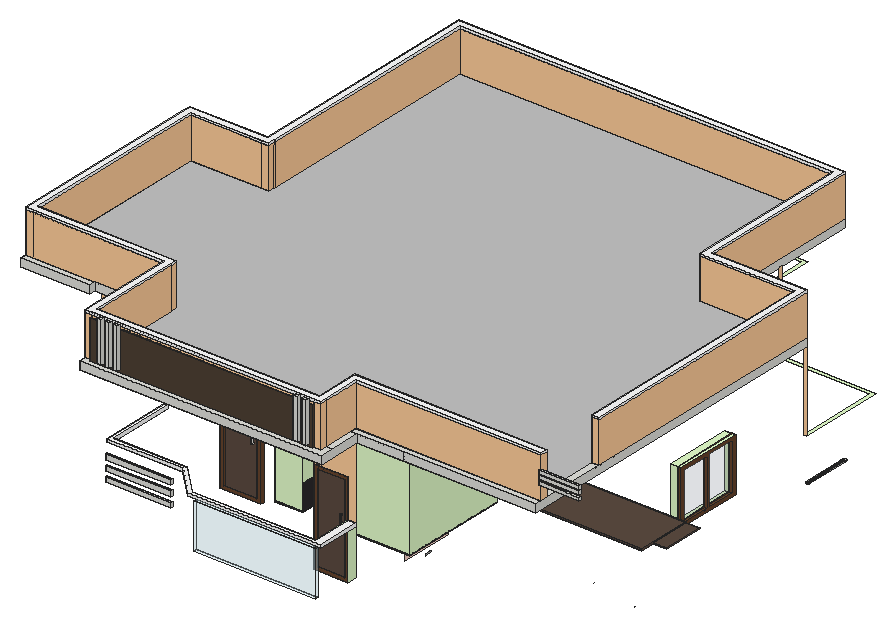
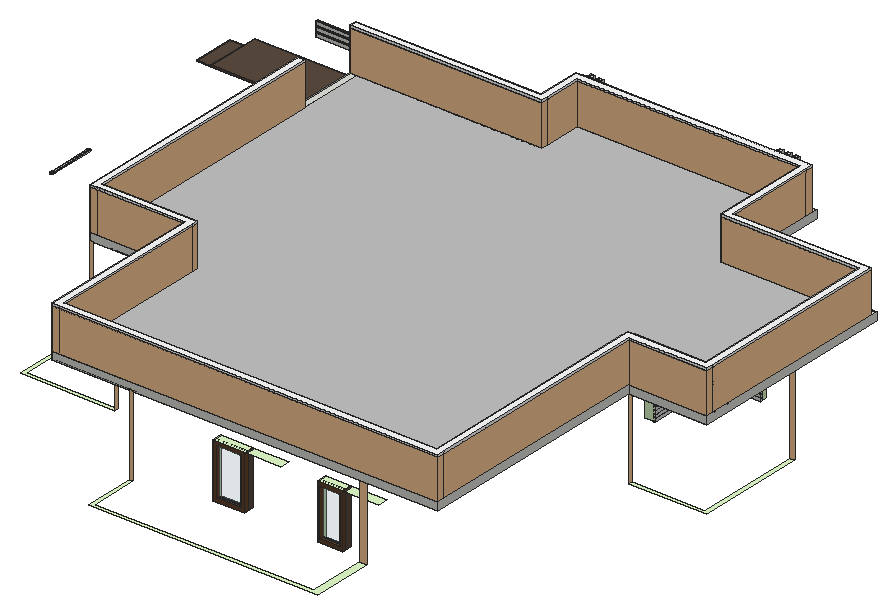
# SketchUp Ruby script. Lengths in inches.
U = 1.inch
M = Sketchup.active_model
def pt(a) = Geom::Point3d.new(a.map { |v| v * U })
def face(e, loops, mat)
  f = e.add_face(loops[0].map { |a| pt(a) })
  loops[1..].each { |l| e.add_face(l.map { |a| pt(a) }).erase! }
  f.material = f.back_material = mat if mat
  f
end
# faces: each face lists its corners as indices into pts; further lists are holes
def faces(e, pts, list, mat = nil) = list.each { |f| face(e, (f[0].is_a?(Array) ? f : [f]).map { |l| l.map { |i| pts[i] } }, mat) }
# xy, xz, yz: faces in a plane at the given z, y or x. An outline is a flat list of corners, or four numbers for a rectangle; further outlines are holes
def ring(l) = l.size == 4 ? [[l[0], l[1]], [l[2], l[1]], [l[2], l[3]], [l[0], l[3]]] : l.each_slice(2).to_a
def flat(e, list, mat, &to3) = list.each { |f| face(e, (f[0].is_a?(Array) ? f : [f]).map { |l| ring(l).map { |u, v| to3.(u, v) } }, mat) }
def xy(e, z, list, mat = nil) = flat(e, list, mat) { |x, y| [x, y, z] }
def xz(e, y, list, mat = nil) = flat(e, list, mat) { |x, z| [x, y, z] }
def yz(e, x, list, mat = nil) = flat(e, list, mat) { |y, z| [x, y, z] }
def lines(e, pts, list) = list.each { |a, b| e.add_line(pt(pts[a]), pt(pts[b])) }
# prism: a flat outline (further loops are holes) pulled along v
def prism(e, loops, v, mat = nil)
  f = face(e, loops, mat); d = Geom::Vector3d.new(v.map { |x| x * U })
  f.pushpull(f.normal.samedirection?(d) ? d.length : -d.length)
end
def box(e, o, s, mat = nil) = prism(e, [[o, [o[0] + s[0], o[1], o[2]], [o[0] + s[0], o[1] + s[1], o[2]], [o[0], o[1] + s[1], o[2]]]], [0, 0, s[2]], mat)
def at(x, y, z, deg = 0) = Geom::Transformation.translation(pt([x, y, z])) * Geom::Transformation.rotation(ORIGIN, Z_AXIS, deg.degrees)
def axes(o, x, y, z) = Geom::Transformation.new([*x, 0, *y, 0, *z, 0, *pt(o).to_a, 1])
def part(name) = M.definitions.add(name)
# library, detail: a bought-in or finely detailed component or shape, given as its bounding box
def library(name, o, s) = part(name).tap { |d| box(d.entities, o, s) }
def detail(e, o, s) = box(e.add_group.entities, o, s)
def put(e, d, t, mat = nil) = e.add_instance(d, t).tap { |i| i.material = mat if mat }
def group(e, t, mat = nil) = e.add_group.tap { |g| g.transformation = t; g.material = mat if mat }.entities
root = M.entities
M.materials.add("Asphalt_01_1K").color = [79, 65, 53]
M.materials.add("B01_Ivory_Dust").color = [255, 217, 206]
M.materials.add("C02_Golden_Beige").color = [255, 205, 155]
M.materials.add("F01_Seafoam_Drift").color = [229, 255, 204]
M.materials.add("Glass_Basic_01").color = [161, 173, 186]
M.materials["Glass_Basic_01"].alpha = 0.25
M.materials.add("Glass_Safety_01").color = [204, 235, 244]
M.materials["Glass_Safety_01"].alpha = 0.25
M.materials.add("M00_Soft_Cloud").color = [255, 255, 255]
M.materials.add("M01_Silver_Fog").color = [224, 224, 224]
M.materials.add("M02_Ash_Whisper").color = [196, 196, 196]
M.materials.add("M03_Pewter_Shine").color = [168, 168, 168]
M.materials.add("M06_Steel_Smoke").color = [86, 86, 86]
M.materials.add("Marble_07_1K").color = [36, 34, 36]
M.materials.add("Metal_06_1K").color = [238, 236, 231]
M.materials.add("Wood_Floor_12_1K").color = [92, 75, 65]
M.materials.add("Wood_Veneer_15_1K").color = [103, 69, 45]
c1 = part("Group\#25")
xy(c1.entities,0,[[0,-3,30,0]],"Wood_Veneer_15_1K")
xy(c1.entities,3,[[3,-2.25,27,0]],"Wood_Floor_12_1K")
xy(c1.entities,3,[[3,-3,27,-2.25]],"Wood_Veneer_15_1K")
xy(c1.entities,81,[[3,-2.25,27,0]],"Wood_Floor_12_1K")
xy(c1.entities,81,[[3,-3,27,-2.25]],"Wood_Veneer_15_1K")
xy(c1.entities,84,[[0,-3,30,0]],"Wood_Veneer_15_1K")
xz(c1.entities,-3,[[[0,0,30,84],[3,3,27,81]]],"Wood_Veneer_15_1K")
xz(c1.entities,-2.25,[[3,3,27,81]],"Wood_Floor_12_1K")
xz(c1.entities,0,[[[0,0,30,84],[3,3,27,81]]],"Wood_Veneer_15_1K")
yz(c1.entities,0,[[-3,0,0,84]],"Wood_Veneer_15_1K")
yz(c1.entities,3,[[-2.25,3,0,81]],"Wood_Floor_12_1K")
yz(c1.entities,3,[[-3,3,-2.25,81]],"Wood_Veneer_15_1K")
yz(c1.entities,27,[[-2.25,3,0,81]],"Wood_Floor_12_1K")
yz(c1.entities,27,[[-3,3,-2.25,81]],"Wood_Veneer_15_1K")
yz(c1.entities,30,[[-3,0,0,84]],"Wood_Veneer_15_1K")
g1 = group(c1.entities,at(22.875,-2.25,50.47),"Metal_06_1K")
xy(g1,-5.5625,[[0,-0.48,1.25,0]],"Metal_06_1K")
xy(g1,-4.9375,[[0,-1.375,1.25,-0.48]],"Metal_06_1K")
xy(g1,-4.6875,[[0,-1.125,1.25,0]],"Metal_06_1K")
xy(g1,-4.6875,[[0,-1.375,1.25,-1.125]],"Wood_Veneer_15_1K")
xy(g1,0,[[0,-1.125,1.25,-0.5],[0,-0.5,1.25,0]],"Metal_06_1K")
xy(g1,0.25,[[0,-1.375,1.25,-1.125],[0,-1.125,1.25,-0.5]],"Metal_06_1K")
xy(g1,0.25,[[0,-0.5,1.25,0]],"Wood_Veneer_15_1K")
xy(g1,1.25,[[0,-0.5,1.25,0]],"Metal_06_1K")
xz(g1,-1.375,[[0,-4.9375,1.25,-4.6875],[0,-4.6875,1.25,0.25]],"Metal_06_1K")
xz(g1,-1.125,[[0,-4.6875,1.25,0],[0,0,1.25,0.25]],"Metal_06_1K")
xz(g1,-0.5,[[0,0.25,1.25,1.25]],"Metal_06_1K")
xz(g1,-0.5,[[0,0,1.25,0.25]],"Wood_Veneer_15_1K")
xz(g1,-0.48,[[0,-5.5625,1.25,-4.9375]],"Metal_06_1K")
xz(g1,0,[[0,0.25,1.25,1.25]],"Metal_06_1K")
xz(g1,0,[[0,-5.5625,1.25,-4.6875],[0,0,1.25,0.25]],"Wood_Veneer_15_1K")
yz(g1,0,[[-0.48,-5.5625,-0.48,-4.9375,-1.375,-4.9375,-1.375,-4.6875,0,-4.6875,0,-5.5625],[-1.375,-4.6875,-1.125,0.25],[-1.125,0,-0.5,0.25],[-0.5,0,0,0.25],[-0.5,0.25,0,1.25]],"Metal_06_1K")
yz(g1,1.25,[[-0.48,-5.5625,0,-5.5625,0,-4.6875,-1.375,-4.6875,-1.375,-4.9375,-0.48,-4.9375],[-1.375,-4.6875,-1.125,0.25],[-1.125,0,-0.5,0.25],[-0.5,0,0,0.25],[-0.5,0.25,0,1.25]],"Metal_06_1K")
c2 = part("Group\#15")
box(c2.entities,[0,0,0],[5.9375,1,0.1875],"M03_Pewter_Shine")
c3 = part("Group\#69")
box(c3.entities,[0,-2,0],[57.75,2,4.3125])
c4 = part("Group\#13")
box(c4.entities,[0,0,0],[1.125,8.25,0.1875],"M03_Pewter_Shine")
c5 = part("Group\#17")
xy(c5.entities,0,[[0,0,1.3125,6.9375]],"M06_Steel_Smoke")
c6 = part("Group\#16")
box(c6.entities,[0,0,0],[1.1875,8,0.25],"M03_Pewter_Shine")
c7 = part("Group\#14")
box(c7.entities,[0,0,0],[5.9375,1,0.1875],"M03_Pewter_Shine")
c8 = part("Group\#12")
box(c8.entities,[0,0,0],[5.9375,1,0.1875],"M03_Pewter_Shine")
c9 = part("Group\#28")
xy(c9.entities,0,[[0,0,28.0625,3]],"Wood_Veneer_15_1K")
xy(c9.entities,3,[[3,0,25.0625,3]],"Wood_Veneer_15_1K")
xy(c9.entities,45,[[3,0,25.0625,3]],"Wood_Veneer_15_1K")
xy(c9.entities,48,[[0,0,28.0625,3]],"Wood_Veneer_15_1K")
xz(c9.entities,0,[[3,3,25.0625,45]],"Glass_Safety_01")
xz(c9.entities,0,[[[0,0,28.0625,48],[3,3,25.0625,45]]],"Wood_Veneer_15_1K")
xz(c9.entities,3,[[[0,0,28.0625,48],[3,3,25.0625,45]]],"Wood_Veneer_15_1K")
yz(c9.entities,0,[[0,0,3,48]],"Wood_Veneer_15_1K")
yz(c9.entities,3,[[0,3,3,45]],"Wood_Veneer_15_1K")
yz(c9.entities,25.0625,[[0,3,3,45]],"Wood_Veneer_15_1K")
yz(c9.entities,28.0625,[[0,0,3,48]],"Wood_Veneer_15_1K")
c10 = part("Group\#27")
xy(c10.entities,0,[[0,0,3,60]],"Wood_Veneer_15_1K")
xy(c10.entities,3,[[0,3,3,29],[0,29,3,31],[0,31,3,57]],"Wood_Veneer_15_1K")
xy(c10.entities,45,[[0,3,3,29],[0,31,3,57]],"Wood_Veneer_15_1K")
xy(c10.entities,48,[[0,0,3,60]],"Wood_Veneer_15_1K")
xz(c10.entities,0,[[0,0,3,48]],"Wood_Veneer_15_1K")
xz(c10.entities,3,[[0,3,3,45]],"Wood_Veneer_15_1K")
xz(c10.entities,29,[[0,3,3,45]],"Wood_Veneer_15_1K")
xz(c10.entities,31,[[0,3,3,45]],"Wood_Veneer_15_1K")
xz(c10.entities,57,[[0,3,3,45]],"Wood_Veneer_15_1K")
xz(c10.entities,60,[[0,0,3,48]],"Wood_Veneer_15_1K")
yz(c10.entities,0,[[3,3,29,45],[31,3,57,45]],"Glass_Basic_01")
yz(c10.entities,0,[[[0,0,60,48],[3,3,57,3,57,45,31,45,31,3,29,3,29,45,3,45]]],"Wood_Veneer_15_1K")
yz(c10.entities,3,[[[0,0,60,48],[3,3,3,45,29,45,29,3,31,3,31,45,57,45,57,3]]],"Wood_Veneer_15_1K")
c11 = part("Group\#29")
xy(c11.entities,0,[[0,0,1,24]])
xy(c11.entities,2.6,[[0,0,1,24]])
xy(c11.entities,3,[[0,0,1,24]])
xy(c11.entities,5.6,[[0,0,1,24]])
xy(c11.entities,6,[[0,0,1,24]])
xy(c11.entities,8.6,[[0,0,1,24]])
xy(c11.entities,9,[[0,0,1,24]])
xy(c11.entities,11.6,[[0,0,1,24]])
xy(c11.entities,12,[[0,0,1,24]])
xy(c11.entities,14.6,[[0,0,1,24]])
xy(c11.entities,15,[[0,0,1,24]])
xy(c11.entities,18,[[0,0,1,24]])
xz(c11.entities,0,[[0,0,1,2.6],[0,3,1,5.6],[0,6,1,8.6],[0,9,1,11.6],[0,12,1,14.6],
  [0,15,1,18]])
xz(c11.entities,24,[[0,0,1,2.6],[0,3,1,5.6],[0,6,1,8.6],[0,9,1,11.6],[0,12,1,14.6],
  [0,15,1,18]])
yz(c11.entities,0,[[0,2.6,24,3],[0,5.6,24,6],[0,8.6,24,9],[0,11.6,24,12],[0,14.6,24,15]])
yz(c11.entities,1,[[0,0,24,2.6],[0,3,24,5.6],[0,6,24,8.6],[0,9,24,11.6],[0,12,24,14.6],
  [0,15,24,18]])
c12 = part("Group\#62")
box(c12.entities,[0,-2.8125,0],[4,2.8125,35.84])
c13 = part("Group\#55")
prism(c13.entities,[[[0,0.5,0],[35.8,0,0],[35.77,-2,0],[-0.03,-1.5,0]]],[0,0,3.01])
prism(root,[[[1692.85,675.6875,154.68],[1801.03,675.6875,154.68],[1801.03,678.6875,154.68],[1797.92,678.6875,154.68],[1692.85,678.6875,154.68]]],[0,0,40.5625],"Glass_Safety_01")
xy(root,150,[[1767.92,714.6875,1797.92,723.6875]],"Wood_Floor_12_1K")
xy(root,184,[[1797.92,723.6875,1797.92,747.03,1797.9375,747.22,1797.97,747.41,1798.04,747.59,1798.08,747.6875,1821.8125,747.6875,1821.8125,819.65,1821.81,819.65,1821.96,819.68,1822.1,819.6875,1845.8125,819.6875,1845.8125,723.6875],[1797.92,747.03,1797.9375,747.22,1797.97,747.41,1798.04,747.59,1798.08,747.6875,1797.92,747.6875]],"B01_Ivory_Dust")
xy(root,184,[[1798.08,747.6875,1798.12,747.76,1798.23,747.92,1798.36,748.07,1798.5,748.2,1798.66,748.3,1798.83,748.39,1799.02,748.45,1799.2,748.49,1799.4,748.5,1821,748.5,1821,747.6875],[1821,747.6875,1821.8125,795.6875],[1821,795.6875,1821,818.59,1821.01,818.73,1821.04,818.87,1821.08,819.01,1821.15,819.14,1821.23,819.26,1821.32,819.37,1821.43,819.46,1821.55,819.54,1821.68,819.6,1821.8125,819.65,1821.8125,795.6875],[1821.81,819.65,1821.96,819.68,1822.1,819.6875,1821.8125,819.6875,1821.8125,819.65]],"Marble_07_1K")
xy(root,185,[[1725.8125,723.6875,1725.8125,819.6875,1748.87,819.6875,1749.1,819.67,1749.32,819.63,1749.54,819.55,1749.75,819.45,1749.8125,819.41,1749.8125,723.73,1749.79,723.73,1749.64,723.7,1749.5,723.6875],[1749.5,723.6875,1749.8125,723.6875,1749.8125,723.73,1749.79,723.73,1749.64,723.7]],"B01_Ivory_Dust")
xy(root,185,[[1959.8125,869.89,1968.8125,929.89],[1651.0625,1117.375,1673.1875,1126.375],[1737.77,1117.375,1765.83,1126.375]],"F01_Seafoam_Drift")
xy(root,185,[[1797.92,723.6875,1845.8125,723.6875,1845.8125,819.6875,1822.1,819.6875,1821.96,819.68,1821.81,819.65,1821.68,819.6,1821.55,819.54,1821.43,819.46,1821.32,819.37,1821.23,819.26,1821.15,819.14,1821.08,819.01,1821.04,818.87,1821.01,818.73,1821,818.59,1821,748.5,1799.4,748.5,1799.2,748.49,1799.02,748.45,1798.83,748.39,1798.66,748.3,1798.5,748.2,1798.36,748.07,1798.23,747.92,1798.12,747.76,1798.04,747.59,1797.97,747.41,1797.9375,747.22,1797.92,747.03],[1749.8125,723.73,1749.8125,747.6875,1750.625,747.6875,1750.625,724.82,1750.62,724.67,1750.59,724.52,1750.54,724.38,1750.47,724.25,1750.39,724.13,1750.29,724.02,1750.18,723.92,1750.06,723.84,1749.93,723.77],[1749.8125,747.6875,1750.625,771.6875],[1749.8125,771.6875,1750.625,795.6875],[1749.8125,795.6875,1749.8125,819.41,1749.9375,819.32,1750.11,819.17,1750.26,819,1750.39,818.81,1750.49,818.6,1750.57,818.38,1750.61,818.16,1750.625,817.93,1750.625,795.6875],
  [1749.8125,819.41,1749.8125,819.6875,1748.87,819.6875,1749.1,819.67,1749.32,819.63,1749.54,819.55,1749.75,819.45]],"Marble_07_1K")
xy(root,186,[[1725.8125,723.6875,1749.5,723.6875,1749.64,723.7,1749.79,723.73,1749.93,723.77,1750.06,723.84,1750.18,723.92,1750.29,724.02,1750.39,724.13,1750.47,724.25,1750.54,724.38,1750.59,724.52,1750.62,724.67,1750.625,724.82,1750.625,817.93,1750.61,818.16,1750.57,818.38,1750.49,818.6,1750.39,818.81,1750.26,819,1750.11,819.17,1749.9375,819.32,1749.75,819.45,1749.54,819.55,1749.32,819.63,1749.1,819.67,1748.87,819.6875,1725.8125,819.6875]],"Marble_07_1K")
xy(root,197,[[1687.27,675.6875,1662.78,700.375,1596.1,700.375,1596.1,763.375,1599.1,763.375,1599.1,703.375,1664.03,703.375,1688.52,678.6875,1797.92,678.6875,1797.92,714.6875,1804.92,714.6875,1804.92,675.6875],[1473.8125,847.375,1477.8125,847.375,1477.8125,941.875,1542.8125,941.875,1542.8125,944.875,1473.8125,944.875],[1965.8125,1009.375,1968.8125,1009.375,1968.8125,1086,1884.8125,1086,1884.8125,1083,1965.8125,1083],[1613.1875,1147.375,1619.1875,1147.375,1619.1875,1198.375,1812.8125,1198.375,1812.8125,1156.375,1815.8125,1156.375,1815.8125,1201.375,1613.1875,1201.375]],"F01_Seafoam_Drift")
xy(root,199.6875,[[1687.27,675.6875,1804.92,675.6875,1804.92,714.6875,1797.92,714.6875,1797.92,678.6875,1688.52,678.6875,1664.03,703.375,1599.1,703.375,1599.1,763.375,1596.1,763.375,1596.1,700.375,1662.78,700.375]],"M00_Soft_Cloud")
xy(root,233,[[1767.92,714.6875,1797.92,723.6875],[1911.8125,763,1959.8125,769],[1645.59,763.375,1681.59,772.375],[1542.8125,811.375,1548.8125,841.375],[1504.12,841.375,1523.47,847.375],
  [1959.8125,869.89,1968.8125,929.89],[1542.8125,897.17,1551.8125,915.375],[1875.8125,1033.59,1884.8125,1057.59],[1619.1875,1117.375,1649.1875,1126.375],[1651.0625,1117.375,1673.1875,1126.375],
  [1705.83,1117.375,1735.83,1126.375],[1737.77,1117.375,1765.83,1126.375]],"F01_Seafoam_Drift")
xy(root,233,[[1649.1875,1117.375,1651.0625,1126.375],[1735.83,1117.375,1737.77,1126.375]],"Wood_Floor_12_1K")
xy(root,233.25,[[1884.8125,1000.375,1920.8125,1009.375]],"F01_Seafoam_Drift")
xy(root,251,[[1504.12,841.375,1523.47,847.375],[1542.8125,897.17,1551.8125,915.375],[1875.8125,1033.59,1884.8125,1057.59]],"F01_Seafoam_Drift")
xy(root,269,[[1716.8125,714.6875,1767.92,714.6875,1767.92,723.6875,1725.8125,723.6875,1725.8125,819.6875,1770.625,819.6875,1770.625,825.6875,1695.8125,825.6875,1695.8125,895.375,1689.8125,895.375,1689.8125,819.6875,1719.8125,819.6875,1719.8125,772.375,1645.59,772.375,1645.59,763.375,1716.8125,763.375],[[1767.92,714.6875,1851.8125,714.6875,1851.8125,763.375,1906.8125,763,1911.8125,763,1911.8125,769,1906.8125,769,1906.8125,825.6875,1806.625,825.6875,1806.625,819.6875,1845.8125,819.6875,1845.8125,723.6875,1767.92,723.6875],[1903.8125,772.02,1851.8125,772.375,1851.8125,822.58,1903.8125,822.63]],[1911.8125,763,1968.8125,763,1968.8125,869.89,1959.8125,869.89,1959.8125,769,1911.8125,769],[1473.8125,763.375,1645.59,763.375,1645.59,772.375,1548.8125,772.375,1548.8125,811.375,1542.8125,811.375,1542.8125,772.375,1482.8125,772.375,1482.8125,841.375,1523.47,841.375,1523.47,847.375,1473.8125,847.375],[1542.8125,811.375,1548.8125,811.375,1548.8125,847.375,1523.47,847.375,1523.47,841.375,1542.8125,841.375],
  [1542.8125,847.375,1548.8125,877.375],[1959.8125,869.89,1968.8125,869.89,1968.8125,1009.375,1920.8125,1009.375,1920.8125,1000.375,1959.8125,1000.375],[1542.8125,877.375,1548.8125,877.375,1548.8125,889.375,1653.8125,889.375,1653.8125,895.375,1551.8125,895.375,1551.8125,915.375,1542.8125,915.375],[1542.8125,915.375,1551.8125,915.375,1551.8125,955.375,1639.8125,955.375,1639.8125,925.375,1645.8125,925.375,1645.8125,961.375,1551.8125,961.375,1551.8125,1141.375,1613.1875,1141.375,1613.1875,1117.375,1619.1875,1117.375,1619.1875,1147.375,1542.8125,1147.375],[1677.8125,945.6875,1683.8125,945.6875,1683.8125,1117.375,1705.83,1117.375,1705.83,1126.375,1619.1875,1126.375,1619.1875,1117.375,1677.8125,1117.375],
  [1719.8125,945.6875,1815.8125,945.6875,1815.8125,1000.375,1920.8125,1000.375,1920.8125,1009.375,1884.8125,1009.375,1884.8125,1033.59,1875.8125,1033.59,1875.8125,1006.375,1815.8125,1006.375,1815.8125,1096.375,1809.8125,1096.375,1809.8125,951.6875,1719.8125,951.6875],[1875.8125,1033.59,1884.8125,1033.59,1884.8125,1156.375,1809.8125,1156.375,1809.8125,1126.375,1705.83,1126.375,1705.83,1117.375,1815.8125,1117.375,1815.8125,1150.375,1875.8125,1150.375,1875.8125,1096.375,1845.8125,1096.375,1845.8125,1090.375,1875.8125,1090.375]],"F01_Seafoam_Drift")
xz(root,675.6875,[[1687.27,197,1804.92,199.6875]],"M00_Soft_Cloud")
xz(root,678.6875,[[1688.52,197,1797.92,199.6875]],"M00_Soft_Cloud")
xz(root,700.375,[[1596.1,197,1662.78,199.6875]],"M00_Soft_Cloud")
xz(root,703.375,[[1599.1,197,1664.03,199.6875]],"M00_Soft_Cloud")
xz(root,714.6875,[[1797.92,199.6875,1804.92,199.6875,1804.92,269,1767.92,269,1767.92,233,1797.92,233]],"C02_Golden_Beige")
xz(root,714.6875,[[1797.92,197,1804.92,199.6875]],"F01_Seafoam_Drift")
xz(root,723.6875,[[1749.5,185,1749.8125,269],[1797.92,185,1797.92,233,1767.92,233,1767.92,269,1845.8125,269,1845.8125,185],[1725.8125,186,1749.5,269]],"F01_Seafoam_Drift")
xz(root,723.6875,[[1797.92,184,1845.8125,185],[1725.8125,185,1749.5,186]],"Marble_07_1K")
xz(root,748.5,[[1799.4,184,1821,185]],"Marble_07_1K")
xz(root,763.375,[[1596.1,199.6875,1599.1,269]],"C02_Golden_Beige")
xz(root,763.375,[[1596.1,197,1599.1,199.6875]],"F01_Seafoam_Drift")
xz(root,769,[[1911.8125,233,1959.8125,269]],"F01_Seafoam_Drift")
xz(root,819.6875,[[1821.8125,184,1822.1,269],[1748.87,185,1749.8125,269],[1822.1,185,1845.8125,269],[1725.8125,186,1748.87,269]],"F01_Seafoam_Drift")
xz(root,819.6875,[[1822.1,184,1845.8125,185],[1725.8125,185,1748.87,186]],"Marble_07_1K")
xz(root,847.375,[[1473.8125,197,1477.8125,269]],"C02_Golden_Beige")
xz(root,869.89,[[1959.8125,185,1968.8125,233]],"F01_Seafoam_Drift")
xz(root,897.17,[[1542.8125,233,1551.8125,251]],"F01_Seafoam_Drift")
xz(root,915.375,[[1542.8125,233,1551.8125,251]],"F01_Seafoam_Drift")
xz(root,929.89,[[1959.8125,185,1968.8125,233]],"F01_Seafoam_Drift")
xz(root,1009.375,[[1965.8125,197,1968.8125,269],[1884.8125,233.25,1920.8125,269]],"C02_Golden_Beige")
xz(root,1033.59,[[1875.8125,233,1884.8125,251]],"F01_Seafoam_Drift")
xz(root,1057.59,[[1875.8125,233,1884.8125,251]],"F01_Seafoam_Drift")
xz(root,1147.375,[[1613.1875,197,1619.1875,269]],"C02_Golden_Beige")
xz(root,1156.375,[[1812.8125,197,1815.8125,269]],"C02_Golden_Beige")
yz(root,1504.12,[[841.375,233,847.375,251]],"F01_Seafoam_Drift")
yz(root,1523.47,[[841.375,233,847.375,251]],"F01_Seafoam_Drift")
yz(root,1542.8125,[[941.875,197,944.875,269]],"C02_Golden_Beige")
yz(root,1542.8125,[[811.375,233,841.375,269]],"F01_Seafoam_Drift")
yz(root,1596.1,[[700.375,197,763.375,199.6875]],"M00_Soft_Cloud")
yz(root,1599.1,[[703.375,197,763.375,199.6875]],"M00_Soft_Cloud")
yz(root,1651.0625,[[1117.375,185,1126.375,233]],"Wood_Floor_12_1K")
yz(root,1673.1875,[[1117.375,185,1126.375,233]],"F01_Seafoam_Drift")
yz(root,1725.8125,[[723.6875,186,819.6875,269]],"F01_Seafoam_Drift")
yz(root,1725.8125,[[723.6875,185,819.6875,186]],"Marble_07_1K")
yz(root,1737.77,[[1117.375,185,1126.375,233]],"Wood_Floor_12_1K")
yz(root,1750.625,[[724.82,185,817.93,186]],"Marble_07_1K")
yz(root,1765.83,[[1117.375,185,1126.375,233]],"F01_Seafoam_Drift")
yz(root,1767.92,[[714.6875,150,723.6875,233]],"F01_Seafoam_Drift")
yz(root,1797.92,[[714.6875,150,723.6875,233],[678.6875,197,714.6875,199.6875]],"F01_Seafoam_Drift")
yz(root,1797.92,[[723.6875,184,747.03,185]],"Marble_07_1K")
yz(root,1804.92,[[675.6875,197,714.6875,199.6875]],"M00_Soft_Cloud")
yz(root,1821,[[748.5,184,818.59,185]],"Marble_07_1K")
yz(root,1821.8125,[[747.6875,161,795.6875,174.875],[747.6875,174.875,795.6875,184]],"B01_Ivory_Dust")
yz(root,1845.8125,[[723.6875,185,819.6875,269]],"F01_Seafoam_Drift")
yz(root,1845.8125,[[723.6875,184,819.6875,185]],"Marble_07_1K")
yz(root,1884.8125,[[1083,197,1086,269]],"C02_Golden_Beige")
yz(root,1920.8125,[[1000.375,233.25,1009.375,269]],"F01_Seafoam_Drift")
p = [[1797.92,747.03,185],[1797.9375,747.22,185],[1797.9375,747.22,184],[1797.92,747.03,184],[1797.97,747.41,185],[1797.97,747.41,184],
  [1798.04,747.59,185],[1798.04,747.59,184],[1798.12,747.76,185],[1798.12,747.76,184],[1798.08,747.6875,184],[1798.23,747.92,185],
  [1798.23,747.92,184],[1798.36,748.07,185],[1798.36,748.07,184],[1798.5,748.2,185],[1798.5,748.2,184],[1798.66,748.3,185],
  [1798.66,748.3,184],[1798.83,748.39,185],[1798.83,748.39,184],[1799.02,748.45,185],[1799.02,748.45,184],[1799.2,748.49,185],
  [1799.2,748.49,184],[1799.4,748.5,185],[1799.4,748.5,184],[1821,818.59,185],[1821.01,818.73,185],[1821.01,818.73,184],
  [1821,818.59,184],[1821.04,818.87,185],[1821.04,818.87,184],[1821.08,819.01,185],[1821.08,819.01,184],[1821.15,819.14,185],
  [1821.15,819.14,184],[1821.23,819.26,185],[1821.23,819.26,184],[1821.32,819.37,185],[1821.32,819.37,184],[1821.43,819.46,185],
  [1821.43,819.46,184],[1821.55,819.54,185],[1821.55,819.54,184],[1821.68,819.6,185],[1821.68,819.6,184],[1821.81,819.65,185],
  [1821.81,819.65,184],[1821.8125,819.65,184],[1821.96,819.68,185],[1821.96,819.68,184],[1822.1,819.6875,185],[1822.1,819.6875,184],
  [1749.64,723.7,186],[1749.5,723.6875,186],[1749.5,723.6875,185],[1749.64,723.7,185],[1749.79,723.73,186],[1749.79,723.73,185],
  [1749.93,723.77,186],[1749.8125,723.73,185],[1749.93,723.77,185],[1750.06,723.84,186],[1750.06,723.84,185],[1750.18,723.92,186],
  [1750.18,723.92,185],[1750.29,724.02,186],[1750.29,724.02,185],[1750.39,724.13,186],[1750.39,724.13,185],[1750.47,724.25,186],
  [1750.47,724.25,185],[1750.54,724.38,186],[1750.54,724.38,185],[1750.59,724.52,186],[1750.59,724.52,185],[1750.62,724.67,186],
  [1750.62,724.67,185],[1750.625,724.82,186],[1750.625,724.82,185],[1750.61,818.16,186],[1750.625,817.93,186],[1750.625,817.93,185],
  [1750.61,818.16,185],[1750.57,818.38,186],[1750.57,818.38,185],[1750.49,818.6,186],[1750.49,818.6,185],[1750.39,818.81,186],
  [1750.39,818.81,185],[1750.26,819,186],[1750.26,819,185],[1750.11,819.17,186],[1750.11,819.17,185],[1749.9375,819.32,186],
  [1749.9375,819.32,185],[1749.75,819.45,186],[1749.8125,819.41,185],[1749.75,819.45,185],[1749.54,819.55,186],[1749.54,819.55,185],
  [1749.1,819.67,186],[1749.32,819.63,186],[1749.32,819.63,185],[1749.1,819.67,185],[1748.87,819.6875,186],[1748.87,819.6875,185],
  [1662.78,700.375,197],[1687.27,675.6875,197],[1687.27,675.6875,199.6875],[1662.78,700.375,199.6875],[1688.52,678.6875,197],[1664.03,703.375,197],
  [1664.03,703.375,199.6875],[1688.52,678.6875,199.6875],[2068.83,923.38,249.1],[2068.83,924.41,249.1],[2069.11,924.7,249],[2069.11,923.38,249],
  [2069.11,884.26,249],[2068.83,884.23,249.1],[2070.01,884.23,249.1],[2069.73,884.26,249],[2069.73,923.38,249],[2069.73,925.31,249],
  [2070.01,925.6,249.1],[2070.01,923.38,249.1],[2069.42,925,248.96],[2069.42,923.38,248.96],[2069.42,884.27,248.96],[2068.58,923.38,249.27],
  [2068.58,924.17,249.27],[2068.58,884.19,249.27],[2070.26,884.19,249.27],[2070.26,925.84,249.27],[2070.26,923.38,249.27],[2068.4,884.14,249.48],
  [2068.4,923.38,249.48],[2068.4,923.98,249.48],[2070.44,884.14,249.48],[2070.44,926.03,249.48],[2070.44,923.38,249.48],[2068.28,923.38,249.73],
  [2068.28,923.86,249.73],[2068.28,884.07,249.73],[2070.5625,884.07,249.73],[2070.5625,926.15,249.73],[2070.5625,923.38,249.73],[2068.24,884,250],
  [2068.24,923.38,250],[2068.24,923.82,250],[2070.6,926.1875,250],[2070.6,923.38,250],[2070.6,884,250],[2068.28,923.38,250.27],
  [2068.28,923.86,250.27],[2068.28,883.9375,250.27],[2070.5625,926.15,250.27],[2070.5625,923.38,250.27],[2070.5625,883.9375,250.27],[2068.4,883.87,250.52],
  [2068.4,923.38,250.52],[2068.4,923.98,250.52],[2070.44,926.03,250.52],[2070.44,923.38,250.52],[2070.44,883.87,250.52],[2068.58,883.82,250.73],
  [2068.58,923.38,250.73],[2068.58,924.17,250.73],[2070.26,883.82,250.73],[2070.26,925.84,250.73],[2070.26,923.38,250.73],[2068.83,883.78,250.9],
  [2068.83,923.38,250.9],[2068.83,924.41,250.9],[2070.01,883.78,250.9],[2070.01,925.6,250.9],[2070.01,923.38,250.9],[2069.11,883.75,251],
  [2069.11,923.38,251],[2069.11,924.7,251],[2069.73,883.75,251],[2069.73,925.31,251],[2069.73,923.38,251],[2069.42,883.74,251.04],
  [2069.42,923.38,251.04],[2069.42,925,251.04],[2003.875,775.63,177],[2003.875,774,177],[1968.8125,774,184],[1968.8125,772.38,184],
  [1765.83,1117.375,233],[1765.83,1117.09,233]]
faces(root,p,[[0,1,2,3],[1,4,5,2],[4,6,7,5],[6,8,9,10,7],[8,11,12,9],[11,13,14,12],[13,15,16,14],[15,17,18,16],
  [17,19,20,18],[19,21,22,20],[21,23,24,22],[23,25,26,24],[27,28,29,30],[28,31,32,29],[31,33,34,32],[33,35,36,34],
  [35,37,38,36],[37,39,40,38],[39,41,42,40],[41,43,44,42],[43,45,46,44],[45,47,48,49,46],[47,50,51,48],[50,52,53,51],
  [54,55,56,57],[58,54,57,59],[60,58,59,61,62],[63,60,62,64],[65,63,64,66],[67,65,66,68],[69,67,68,70],[71,69,70,72],
  [73,71,72,74],[75,73,74,76],[77,75,76,78],[79,77,78,80],[81,82,83,84],[85,81,84,86],[87,85,86,88],[89,87,88,90],
  [91,89,90,92],[93,91,92,94],[95,93,94,96],[97,95,96,98,99],[100,97,99,101],[102,103,104,105],[103,100,101,104],[106,102,105,107]],"Marble_07_1K")
faces(root,p,[[108,109,110,111],[112,113,114,115]],"M00_Soft_Cloud")
faces(root,p,[[116,117,118,119,120,121],[122,123,124,125,126,127],[119,118,128,129,130,120],[129,128,125,124,123,130],[131,132,117,116,121,133],[134,122,127,126,135,136],[133,137,138,139,132,131],[140,134,136,135,141,142],
  [143,144,139,138,137,145],[146,140,142,141,147,148],[145,149,150,151,144,143],[148,147,152,153,154,146],[155,156,151,150,149,157],[153,152,158,159,160,154],[157,161,162,163,156,155],[159,158,164,165,166,160],
  [161,167,168,169,163,162],[170,166,165,164,171,172],[167,173,174,175,169,168],[176,170,172,171,177,178],[173,179,180,181,175,174],[182,176,178,177,183,184],[179,185,186,187,181,180],[185,182,184,183,187,186]])
lines(root,p,[[188,189],[190,191],[192,193]])
put(root,c1,at(1767.92,717.6875,150),"C02_Golden_Beige")
put(root,c1,axes([1645.59,766.375,150],[1.2,0,0],[0,1,0],[0,0,1]),"C02_Golden_Beige")
put(root,c2,axes([1821.8125,776.71,155.33],[0,-1,0],[0,0,1],[-1,0,0]),"M03_Pewter_Shine")
put(root,c3,at(1596.1,700.375,165.79))
put(root,c4,axes([1821.8125,799.69,166.9],[0,-1,0],[0,0,1],[-1,0,0]),"C02_Golden_Beige")
put(root,c5,axes([1749.8125,743.625,167.35],[0,1,0],[0,0,1],[1,0,0]),"M06_Steel_Smoke")
put(root,c5,axes([1749.8125,749.3125,167.35],[0,1,0],[0,0,1],[1,0,0]),"M06_Steel_Smoke")
put(root,c5,axes([1749.8125,774.25,167.35],[0,1,0],[0,0,1],[1,0,0]),"M06_Steel_Smoke")
put(root,c5,axes([1749.8125,768.5625,167.35],[0,1,0],[0,0,1],[1,0,0]),"M06_Steel_Smoke")
put(root,c5,axes([1749.8125,792.5625,167.35],[0,1,0],[0,0,1],[1,0,0]),"M06_Steel_Smoke")
put(root,c5,axes([1749.8125,798.25,167.35],[0,1,0],[0,0,1],[1,0,0]),"M06_Steel_Smoke")
put(root,c6,axes([1819.5,747.6875,167.4],[-1,0,0],[0,0,1],[0,1,0]),"C02_Golden_Beige")
put(root,c7,axes([1821.8125,776.71,168.14],[0,-1,0],[0,0,1],[-1,0,0]),"M03_Pewter_Shine")
put(root,c3,at(1596.1,700.375,174.79))
put(root,c8,axes([1821.8125,776.71,180.83],[0,-1,0],[0,0,1],[-1,0,0]),"M03_Pewter_Shine")
put(root,c3,at(1596.1,700.375,183.79))
put(root,c9,at(1737.77,1123.375,185),"C02_Golden_Beige")
put(root,c10,at(1965.8125,869.89,185),"C02_Golden_Beige")
put(root,c9,axes([1651.0625,1123.375,185],[0.78842,0,0],[0,1,0],[0,0,1]),"C02_Golden_Beige")
put(root,c11,axes([1523.45,846.375,233],[0,1,0],[-0.8056,0,0],[0,0,1]),"M01_Silver_Fog")
put(root,c11,at(1883.8125,1033.59,233),"M01_Silver_Fog")
put(root,c11,axes([1543.8125,915.37,233],[-1,0,0],[0,-0.76,0],[0,0,1]),"M01_Silver_Fog")
g2 = group(root,at(1851.8125,714.6875,268),"Wood_Floor_12_1K")
xy(g2,-1,[[0,0,206.65,48.32]])
xy(g2,0.0625,[[0,0,206.65,48.32]])
xz(g2,0,[[0,-1,206.65,0.0625]])
xz(g2,48.32,[[0,-1,206.65,0.0625]])
yz(g2,0,[[0,-1,48.32,0.0625]])
yz(g2,206.65,[[0,-1,12.08,-1,12.08,0,48.32,0,48.32,0.0625,0,0.0625]])
p = [[206.65,12,-1],[206.65,12,0]]
lines(g2,p,[[0,1]])
g3 = group(g2,at(206.65,12.08,-1))
box(g3,[0,0,0],[12,36.24,1])
g4 = group(root,at(1542.8125,762.63,269))
xy(g4,-1,[[53.28,-92.95,53.28,0.37,-7.86,0.37,-7.86,-5.63,-69,-5.63,-69,181.87,0,181.87,0,393.37,342,393.37,342,246.37,426,246.37,426,-53.95,268.1,-53.95,268.1,-92.95]],"Wood_Floor_12_1K")
xy(g4,6,[[53.28,-92.95,268.1,-92.95,268.1,-80.95,59.28,-80.95,59.28,6.37,-63,6.37,-63,175.87,6,175.87,6,387.37,336,387.37,336,240.37,420,240.37,420,15.66,426,15.66,426,246.37,342,246.37,342,393.37,0,393.37,0,181.87,-69,181.87,-69,-5.63,-7.86,-5.63,-7.86,0.37,53.28,0.37],[256.1,-80.95,268.1,-80.95,268.1,-53.95,262.1,-53.95,262.1,-41.95,256.1,-41.95],[262.1,-53.95,426,-41.95],[420,-41.95,426,15.66]])
xy(g4,6,[[59.28,-80.95,256.1,-80.95,256.1,-41.95,420,-41.95,420,240.37,336,240.37,336,387.37,6,387.37,6,175.87,-63,175.87,-63,6.37,59.28,6.37]],"M02_Ash_Whisper")
xz(g4,-92.95,[[53.28,-1,268.1,6]])
xz(g4,-53.95,[[268.1,-1,309,6],[309,-1,426,6]])
xz(g4,-5.63,[[-69,-1,-7.86,6]])
xz(g4,0.37,[[-7.86,-1,53.28,6]])
xz(g4,181.87,[[-69,-1,0,6]])
xz(g4,246.37,[[342,-1,426,6]])
xz(g4,393.37,[[0,-1,342,6]])
yz(g4,-69,[[-5.63,-1,181.87,6]])
yz(g4,-7.86,[[-5.63,-1,0.37,6]])
yz(g4,0,[[181.87,-1,393.37,6]])
yz(g4,53.28,[[-92.95,-1,0.37,6]])
yz(g4,268.1,[[-92.95,-1,-53.95,6]])
yz(g4,342,[[246.37,-1,393.37,6]])
yz(g4,426,[[-53.95,-1,246.37,6]])
g5 = group(root,at(1602.1,675.6875,275),"C02_Golden_Beige")
xy(g5,0,[[-6,0,0,6],[0,0,196.82,6],[196.82,0,202.82,6],[-6,6,0,87.32],[196.82,6,202.82,39],
  [196.82,39,366.72,45],[-128.28,87.32,-122.28,262.82],[-122.28,87.32,0,93.32],[360.72,102.88,366.72,333.32],[-128.28,262.82,-59.28,268.82],
  [-59.28,262.82,-53.28,268.69],[-59.28,268.69,-53.28,268.82],[-59.28,268.82,-53.28,474.32],[276.72,327.32,360.72,333.32],[276.72,333.32,282.72,480.32],
  [-59.28,474.32,276.72,480.32]])
xy(g5,36,[[-6,0,-6,87.32,-128.28,87.32,-128.28,268.82,-59.28,268.82,-59.28,480.32,282.72,480.32,282.72,333.32,366.72,333.32,366.72,102.88,360.72,102.88,360.72,327.32,276.72,327.32,276.72,474.32,-53.28,474.32,-53.28,262.82,-122.28,262.82,-122.28,93.32,0,93.32,0,6,196.82,6,196.82,45,366.72,45,366.72,39,202.82,39,202.82,0]],"M00_Soft_Cloud")
xy(g5,37.9375,[[-6,0,202.82,0,202.82,39,366.72,39,366.72,45,196.82,45,196.82,6,0,6,0,93.32,-122.28,93.32,-122.28,262.82,-53.28,262.82,-53.28,474.32,276.72,474.32,276.72,327.32,360.72,327.32,360.72,102.88,366.72,102.88,366.72,333.32,282.72,333.32,282.72,480.32,-59.28,480.32,-59.28,268.82,-128.28,268.82,-128.28,87.32,-6,87.32]],"M00_Soft_Cloud")
xz(g5,0,[[-6,0,0,36],[0,0,196.82,36],[196.82,0,202.82,36]])
xz(g5,0,[[-6,36,0,37.9375],[0,36,196.82,37.9375],[196.82,36,202.82,37.9375]],"M00_Soft_Cloud")
xz(g5,6,[[0,0,196.82,36]])
xz(g5,6,[[0,36,196.82,37.9375]],"M00_Soft_Cloud")
xz(g5,39,[[202.82,0,366.72,36]])
xz(g5,39,[[202.82,36,366.72,37.9375]],"M00_Soft_Cloud")
xz(g5,45,[[196.82,0,366.72,36]])
xz(g5,45,[[196.82,36,366.72,37.9375]],"M00_Soft_Cloud")
xz(g5,87.32,[[-128.28,0,-122.28,36],[-122.28,0,-6,36]])
xz(g5,87.32,[[-128.28,36,-122.28,37.9375],[-122.28,36,-6,37.9375]],"M00_Soft_Cloud")
xz(g5,93.32,[[-122.28,0,0,36]])
xz(g5,93.32,[[-122.28,36,0,37.9375]],"M00_Soft_Cloud")
xz(g5,102.88,[[360.72,0,366.72,36]])
xz(g5,102.88,[[360.72,36,366.72,37.9375]],"M00_Soft_Cloud")
xz(g5,262.82,[[-122.28,0,-59.28,36],[-59.28,0,-53.28,36]])
xz(g5,262.82,[[-122.28,36,-59.28,37.9375],[-59.28,36,-53.28,37.9375]],"M00_Soft_Cloud")
xz(g5,268.82,[[-128.28,0,-59.28,36]])
xz(g5,268.82,[[-128.28,36,-59.28,37.9375]],"M00_Soft_Cloud")
xz(g5,327.32,[[276.72,0,360.72,36]])
xz(g5,327.32,[[276.72,36,360.72,37.9375]],"M00_Soft_Cloud")
xz(g5,333.32,[[282.72,0,360.72,36],[360.72,0,366.72,36]])
xz(g5,333.32,[[282.72,36,360.72,37.9375],[360.72,36,366.72,37.9375]],"M00_Soft_Cloud")
xz(g5,474.32,[[-53.28,0,276.72,36]])
xz(g5,474.32,[[-53.28,36,276.72,37.9375]],"M00_Soft_Cloud")
xz(g5,480.32,[[-59.28,0,276.72,36],[276.72,0,282.72,36]])
xz(g5,480.32,[[-59.28,36,276.72,37.9375],[276.72,36,282.72,37.9375]],"M00_Soft_Cloud")
yz(g5,-128.28,[[87.32,0,262.82,36],[262.82,0,268.82,36]])
yz(g5,-128.28,[[87.32,36,262.82,37.9375],[262.82,36,268.82,37.9375]],"M00_Soft_Cloud")
yz(g5,-122.28,[[93.32,0,262.82,36]])
yz(g5,-122.28,[[93.32,36,262.82,37.9375]],"M00_Soft_Cloud")
yz(g5,-59.28,[[268.69,0,268.82,36],[268.82,0,474.32,36],[474.32,0,480.32,36]])
yz(g5,-59.28,[[268.82,36,474.32,37.9375],[474.32,36,480.32,37.9375]],"M00_Soft_Cloud")
yz(g5,-53.28,[[262.82,0,268.69,36],[268.69,0,268.82,36],[268.82,0,474.32,36]])
yz(g5,-53.28,[[262.82,36,268.69,37.9375],[268.69,36,268.82,37.9375],[268.82,36,474.32,37.9375]],"M00_Soft_Cloud")
yz(g5,-6,[[0,0,6,36],[6,0,87.32,36]])
yz(g5,-6,[[0,36,6,37.9375],[6,36,87.32,37.9375]],"M00_Soft_Cloud")
yz(g5,0,[[6,0,87.32,36],[87.32,0,93.32,36]])
yz(g5,0,[[6,36,87.32,37.9375],[87.32,36,93.32,37.9375]],"M00_Soft_Cloud")
yz(g5,196.82,[[6,0,39,36],[39,0,45,36]])
yz(g5,196.82,[[6,36,39,37.9375],[39,36,45,37.9375]],"M00_Soft_Cloud")
yz(g5,202.82,[[0,0,6,36],[6,0,39,36]])
yz(g5,202.82,[[0,36,6,37.9375],[6,36,39,37.9375]],"M00_Soft_Cloud")
yz(g5,276.72,[[327.32,0,333.32,36],[333.32,0,474.32,36]])
yz(g5,276.72,[[327.32,36,333.32,37.9375],[333.32,36,474.32,37.9375]],"M00_Soft_Cloud")
yz(g5,282.72,[[333.32,0,480.32,36]])
yz(g5,282.72,[[333.32,36,480.32,37.9375]],"M00_Soft_Cloud")
yz(g5,360.72,[[102.88,0,327.32,36]])
yz(g5,360.72,[[102.88,36,327.32,37.9375]],"M00_Soft_Cloud")
yz(g5,366.72,[[39,0,45,36],[102.88,0,333.32,36]])
yz(g5,366.72,[[39,36,45,37.9375],[102.88,36,333.32,37.9375]],"M00_Soft_Cloud")
g6 = group(root,at(1602.1,675.6875,275))
box(g6,[0,-1.625,0],[196.82,1.625,33.85],"Asphalt_01_1K")
g7 = group(root,at(1610.15,674.0625,277.1))
box(g7,[0,-2.8125,0],[4,2.8125,35.84])
g8 = group(root,at(1617.09,674.0625,277.1))
box(g8,[0,-2.8125,0],[4,2.8125,35.84])
put(root,c12,at(1624.03,674.0625,277.1))
put(root,c12,at(1791.65,674.0625,277.1))
put(root,c12,at(1784.15,674.0625,277.1))
put(root,c13,at(1968.8125,714.1875,288.19))
put(root,c13,at(1968.8125,714.1875,293.07))
put(root,c13,at(1968.8125,714.1875,297.44))
